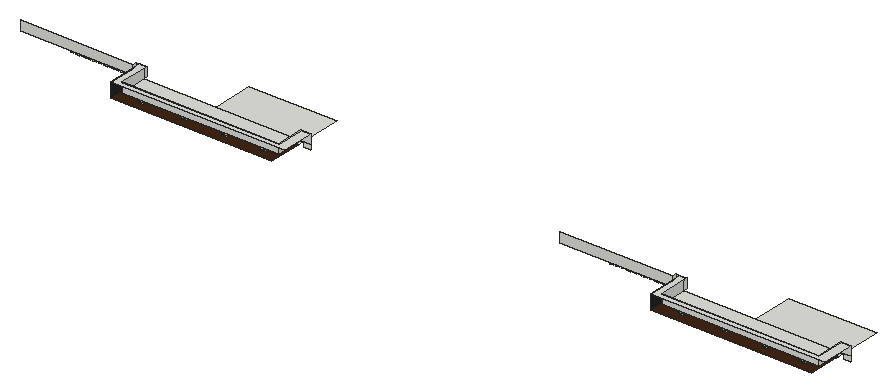
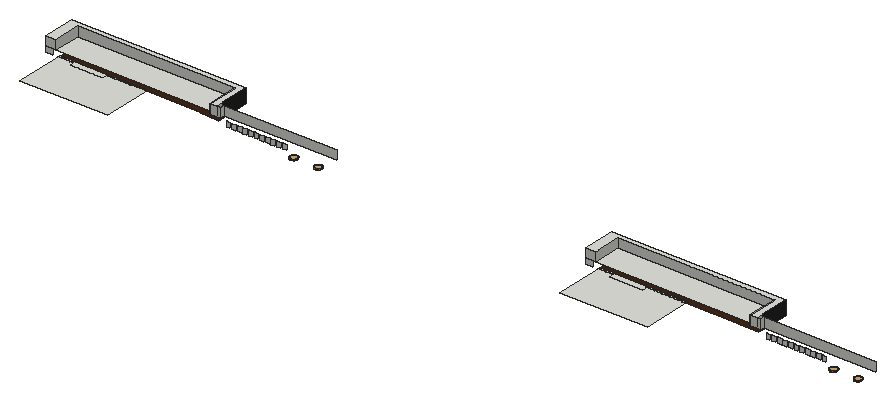
# SketchUp Ruby script. Lengths in inches.
U = 1.inch
M = Sketchup.active_model
def pt(a) = Geom::Point3d.new(a.map { |v| v * U })
def face(e, loops, mat)
  f = e.add_face(loops[0].map { |a| pt(a) })
  loops[1..].each { |l| e.add_face(l.map { |a| pt(a) }).erase! }
  f.material = f.back_material = mat if mat
  f
end
# faces: each face lists its corners as indices into pts; further lists are holes
def faces(e, pts, list, mat = nil) = list.each { |f| face(e, (f[0].is_a?(Array) ? f : [f]).map { |l| l.map { |i| pts[i] } }, mat) }
# xy, xz, yz: faces in a plane at the given z, y or x. An outline is a flat list of corners, or four numbers for a rectangle; further outlines are holes
def ring(l) = l.size == 4 ? [[l[0], l[1]], [l[2], l[1]], [l[2], l[3]], [l[0], l[3]]] : l.each_slice(2).to_a
def flat(e, list, mat, &to3) = list.each { |f| face(e, (f[0].is_a?(Array) ? f : [f]).map { |l| ring(l).map { |u, v| to3.(u, v) } }, mat) }
def xy(e, z, list, mat = nil) = flat(e, list, mat) { |x, y| [x, y, z] }
def xz(e, y, list, mat = nil) = flat(e, list, mat) { |x, z| [x, y, z] }
def yz(e, x, list, mat = nil) = flat(e, list, mat) { |y, z| [x, y, z] }
def lines(e, pts, list) = list.each { |a, b| e.add_line(pt(pts[a]), pt(pts[b])) }
# prism: a flat outline (further loops are holes) pulled along v
def prism(e, loops, v, mat = nil)
  f = face(e, loops, mat); d = Geom::Vector3d.new(v.map { |x| x * U })
  f.pushpull(f.normal.samedirection?(d) ? d.length : -d.length)
end
def box(e, o, s, mat = nil) = prism(e, [[o, [o[0] + s[0], o[1], o[2]], [o[0] + s[0], o[1] + s[1], o[2]], [o[0], o[1] + s[1], o[2]]]], [0, 0, s[2]], mat)
def at(x, y, z, deg = 0) = Geom::Transformation.translation(pt([x, y, z])) * Geom::Transformation.rotation(ORIGIN, Z_AXIS, deg.degrees)
def axes(o, x, y, z) = Geom::Transformation.new([*x, 0, *y, 0, *z, 0, *pt(o).to_a, 1])
def part(name) = M.definitions.add(name)
# library, detail: a bought-in or finely detailed component or shape, given as its bounding box
def library(name, o, s) = part(name).tap { |d| box(d.entities, o, s) }
def detail(e, o, s) = box(e.add_group.entities, o, s)
def put(e, d, t, mat = nil) = e.add_instance(d, t).tap { |i| i.material = mat if mat }
def group(e, t, mat = nil) = e.add_group.tap { |g| g.transformation = t; g.material = mat if mat }.entities
root = M.entities
M.materials.add("[Field Square Tile]").color = [211, 167, 108]
M.materials.add("[Granite Dark Gray]").color = [38, 37, 37]
M.materials.add("[Wood Veneer 01]").color = [66, 38, 20]
xy(root,380.5,[[2291.96,508.33,2297.38,511.08],[2297.38,508.33,2298.58,511.08],[2298.58,508.33,2304.01,511.08],[2304.01,508.33,2305.21,511.08],[2305.21,508.33,2310.63,511.08],
  [2310.63,508.33,2311.83,511.08],[2311.83,508.33,2317.26,511.08],[2317.26,508.33,2318.46,511.08],[2318.46,508.33,2323.88,511.08],[2323.88,508.33,2325.08,511.08],
  [2325.08,508.33,2330.51,511.08],[2330.51,508.33,2331.71,511.08],[2331.71,508.33,2337.13,511.08],[2337.13,508.33,2338.33,511.08],[2338.33,508.33,2343.76,511.08],
  [2343.76,508.33,2344.96,511.08],[2344.96,508.33,2350.38,511.08],[2350.38,508.33,2351.58,511.08],[2351.58,508.33,2357.01,511.08],[2357.01,508.33,2410.56,518.65],
  [2410.56,508.33,2415.98,511.08],[2415.98,508.33,2417.18,511.08],[2417.18,508.33,2422.61,511.08],[2422.61,508.33,2423.81,511.08],[2423.81,508.33,2429.23,511.08],
  [2429.23,508.33,2430.06,511.08],[2430.06,508.33,2434.04,511.08],[2434.04,508.33,2435.48,511.08],[3170.71,508.33,3176.13,511.08],[3176.13,508.33,3177.33,511.08],
  [3177.33,508.33,3182.76,511.08],[3182.76,508.33,3183.96,511.08],[3183.96,508.33,3189.38,511.08],[3189.38,508.33,3190.58,511.08],[3190.58,508.33,3196.01,511.08],
  [3196.01,508.33,3197.21,511.08],[3197.21,508.33,3202.63,511.08],[3202.63,508.33,3203.83,511.08],[3203.83,508.33,3209.26,511.08],[3209.26,508.33,3210.46,511.08],
  [3210.46,508.33,3215.88,511.08],[3215.88,508.33,3217.08,511.08],[3217.08,508.33,3222.51,511.08],[3222.51,508.33,3223.71,511.08],[3223.71,508.33,3229.13,511.08],
  [3229.13,508.33,3230.33,511.08],[3230.33,508.33,3235.76,511.08],[3235.76,508.33,3289.31,518.65],[3289.31,508.33,3294.73,511.08],[3294.73,508.33,3295.93,511.08],
  [3295.93,508.33,3301.36,511.08],[3301.36,508.33,3302.56,511.08],[3302.56,508.33,3307.98,511.08],[3307.98,508.33,3308.81,511.08],[3308.81,508.33,3312.79,511.08],
  [3312.79,508.33,3314.23,511.08],[2291.96,511.08,2291.96,589.83,2434.04,589.83,2434.04,511.08,2410.56,511.08,2410.56,518.65,2357.01,518.65,2357.01,511.08],[3170.71,511.08,3170.71,589.83,3312.79,589.83,3312.79,511.08,3289.31,511.08,3289.31,518.65,3235.76,518.65,3235.76,511.08]])
xy(root,380.5,[[[2172.48,458.5,2172.48,512.27,2202.28,512.27,2202.28,511.08,2291.96,511.08,2291.96,508.33,2434.04,508.33,2434.04,458.5],[2279.18,470.7,2280.73,470.9,2282.18,471.5,2283.42,472.46,2284.38,473.7,2284.98,475.15,2285.18,476.7,2284.98,478.25,2284.38,479.7,2283.42,480.94,2282.18,481.9,2280.73,482.49,2279.18,482.7,2277.63,482.49,2276.18,481.9,2274.9375,480.94,2273.99,479.7,2273.39,478.25,2273.18,476.7,2273.39,475.15,2273.99,473.7,2274.9375,472.46,2276.18,471.5,2277.63,470.9],[2346.46,470.7,2348.01,470.9,2349.46,471.5,2350.7,472.46,2351.66,473.7,2352.26,475.15,2352.46,476.7,2352.26,478.25,2351.66,479.7,2350.7,480.94,2349.46,481.9,2348.01,482.49,2346.46,482.7,2344.91,482.49,2343.46,481.9,2342.22,480.94,2341.26,479.7,2340.66,478.25,2340.46,476.7,2340.66,475.15,2341.26,473.7,2342.22,472.46,2343.46,471.5,2344.91,470.9],[2407.83,470.7,2409.39,470.9,2410.83,471.5,2412.08,472.46,2413.03,473.7,2413.63,475.15,2413.83,476.7,2413.63,478.25,2413.03,479.7,2412.08,480.94,2410.83,481.9,2409.39,482.49,2407.83,482.7,2406.28,482.49,2404.83,481.9,2403.59,480.94,2402.64,479.7,2402.04,478.25,2401.83,476.7,2402.04,475.15,2402.64,473.7,2403.59,472.46,2404.83,471.5,2406.28,470.9],[2209.72,470.7,2211.27,470.9,2212.72,471.5,2213.96,472.46,2214.91,473.7,2215.51,475.15,2215.72,476.7,2215.51,478.25,2214.91,479.7,2213.96,480.94,2212.72,481.9,2211.27,482.49,2209.72,482.7,2208.17,482.49,2206.72,481.9,2205.48,480.94,2204.52,479.7,2203.92,478.25,2203.72,476.7,2203.92,475.15,2204.52,473.7,2205.48,472.46,2206.72,471.5,2208.17,470.9]],[[3051.23,458.5,3051.23,512.27,3081.03,512.27,3081.03,511.08,3170.71,511.08,3170.71,508.33,3312.79,508.33,3312.79,458.5],[3157.93,470.7,3159.48,470.9,3160.93,471.5,3162.17,472.46,3163.13,473.7,3163.73,475.15,3163.93,476.7,3163.73,478.25,3163.13,479.7,3162.17,480.94,3160.93,481.9,3159.48,482.49,3157.93,482.7,3156.38,482.49,3154.93,481.9,3153.6875,480.94,3152.74,479.7,3152.14,478.25,3151.93,476.7,3152.14,475.15,3152.74,473.7,3153.6875,472.46,3154.93,471.5,3156.38,470.9],[3286.58,470.7,3288.14,470.9,3289.58,471.5,3290.83,472.46,3291.78,473.7,3292.38,475.15,3292.58,476.7,3292.38,478.25,3291.78,479.7,3290.83,480.94,3289.58,481.9,3288.14,482.49,3286.58,482.7,3285.03,482.49,3283.58,481.9,3282.34,480.94,3281.39,479.7,3280.79,478.25,3280.58,476.7,3280.79,475.15,3281.39,473.7,3282.34,472.46,3283.58,471.5,3285.03,470.9],[3088.47,470.7,3090.02,470.9,3091.47,471.5,3092.71,472.46,3093.66,473.7,3094.26,475.15,3094.47,476.7,3094.26,478.25,3093.66,479.7,3092.71,480.94,3091.47,481.9,3090.02,482.49,3088.47,482.7,3086.92,482.49,3085.47,481.9,3084.23,480.94,3083.27,479.7,3082.67,478.25,3082.47,476.7,3082.67,475.15,3083.27,473.7,3084.23,472.46,3085.47,471.5,3086.92,470.9],[3225.21,470.7,3226.76,470.9,3228.21,471.5,3229.45,472.46,3230.41,473.7,3231.01,475.15,3231.21,476.7,3231.01,478.25,3230.41,479.7,3229.45,480.94,3228.21,481.9,3226.76,482.49,3225.21,482.7,3223.66,482.49,3222.21,481.9,3220.97,480.94,3220.01,479.7,3219.41,478.25,3219.21,476.7,3219.41,475.15,3220.01,473.7,3220.97,472.46,3222.21,471.5,3223.66,470.9]]],"[Wood Veneer 01]")
xy(root,381.8125,[[2209.72,470.7,2208.17,470.9,2206.72,471.5,2205.48,472.46,2204.52,473.7,2203.92,475.15,2203.72,476.7,2203.92,478.25,2204.52,479.7,2205.48,480.94,2206.72,481.9,2208.17,482.49,2209.72,482.7,2211.27,482.49,2212.72,481.9,2213.96,480.94,2214.91,479.7,2215.51,478.25,2215.72,476.7,2215.51,475.15,2214.91,473.7,2213.96,472.46,2212.72,471.5,2211.27,470.9],[2279.18,470.7,2277.63,470.9,2276.18,471.5,2274.9375,472.46,2273.99,473.7,2273.39,475.15,2273.18,476.7,2273.39,478.25,2273.99,479.7,2274.9375,480.94,2276.18,481.9,2277.63,482.49,2279.18,482.7,2280.73,482.49,2282.18,481.9,2283.42,480.94,2284.38,479.7,2284.98,478.25,2285.18,476.7,2284.98,475.15,2284.38,473.7,2283.42,472.46,2282.18,471.5,2280.73,470.9],[2346.46,470.7,2344.91,470.9,2343.46,471.5,2342.22,472.46,2341.26,473.7,2340.66,475.15,2340.46,476.7,2340.66,478.25,2341.26,479.7,2342.22,480.94,2343.46,481.9,2344.91,482.49,2346.46,482.7,2348.01,482.49,2349.46,481.9,2350.7,480.94,2351.66,479.7,2352.26,478.25,2352.46,476.7,2352.26,475.15,2351.66,473.7,2350.7,472.46,2349.46,471.5,2348.01,470.9],[2407.83,470.7,2406.28,470.9,2404.83,471.5,2403.59,472.46,2402.64,473.7,2402.04,475.15,2401.83,476.7,2402.04,478.25,2402.64,479.7,2403.59,480.94,2404.83,481.9,2406.28,482.49,2407.83,482.7,2409.39,482.49,2410.83,481.9,2412.08,480.94,2413.03,479.7,2413.63,478.25,2413.83,476.7,2413.63,475.15,2413.03,473.7,2412.08,472.46,2410.83,471.5,2409.39,470.9],[3088.47,470.7,3086.92,470.9,3085.47,471.5,3084.23,472.46,3083.27,473.7,3082.67,475.15,3082.47,476.7,3082.67,478.25,3083.27,479.7,3084.23,480.94,3085.47,481.9,3086.92,482.49,3088.47,482.7,3090.02,482.49,3091.47,481.9,3092.71,480.94,3093.66,479.7,3094.26,478.25,3094.47,476.7,3094.26,475.15,3093.66,473.7,3092.71,472.46,3091.47,471.5,3090.02,470.9],
  [3157.93,470.7,3156.38,470.9,3154.93,471.5,3153.6875,472.46,3152.74,473.7,3152.14,475.15,3151.93,476.7,3152.14,478.25,3152.74,479.7,3153.6875,480.94,3154.93,481.9,3156.38,482.49,3157.93,482.7,3159.48,482.49,3160.93,481.9,3162.17,480.94,3163.13,479.7,3163.73,478.25,3163.93,476.7,3163.73,475.15,3163.13,473.7,3162.17,472.46,3160.93,471.5,3159.48,470.9],[3225.21,470.7,3223.66,470.9,3222.21,471.5,3220.97,472.46,3220.01,473.7,3219.41,475.15,3219.21,476.7,3219.41,478.25,3220.01,479.7,3220.97,480.94,3222.21,481.9,3223.66,482.49,3225.21,482.7,3226.76,482.49,3228.21,481.9,3229.45,480.94,3230.41,479.7,3231.01,478.25,3231.21,476.7,3231.01,475.15,3230.41,473.7,3229.45,472.46,3228.21,471.5,3226.76,470.9],[3286.58,470.7,3285.03,470.9,3283.58,471.5,3282.34,472.46,3281.39,473.7,3280.79,475.15,3280.58,476.7,3280.79,478.25,3281.39,479.7,3282.34,480.94,3283.58,481.9,3285.03,482.49,3286.58,482.7,3288.14,482.49,3289.58,481.9,3290.83,480.94,3291.78,479.7,3292.38,478.25,3292.58,476.7,3292.38,475.15,3291.78,473.7,3290.83,472.46,3289.58,471.5,3288.14,470.9]],"[Field Square Tile]")
xy(root,381.875,[[1998.33,523.51,1996.77,523.54,1995.26,523.98,1993.92,524.79,1992.84,525.92,1992.08,527.29,1991.71,528.8125,1991.74,530.375,1992.18,531.88,1992.99,533.22,1994.12,534.31,1995.49,535.06,1997.01,535.43,1998.58,535.4,2000.08,534.96,2001.42,534.15,2002.51,533.02,2003.26,531.65,2003.64,530.13,2003.6,528.5625,2003.17,527.06,2002.36,525.72,2001.23,524.64,1999.85,523.88],[2038.08,523.51,2036.52,523.54,2035.01,523.98,2033.67,524.79,2032.59,525.92,2031.83,527.29,2031.46,528.8125,2031.49,530.375,2031.93,531.88,2032.74,533.22,2033.87,534.31,2035.24,535.06,2036.76,535.43,2038.33,535.4,2039.83,534.96,2041.17,534.15,2042.26,533.02,2043.01,531.65,2043.39,530.13,2043.35,528.5625,2042.92,527.06,2042.11,525.72,2040.98,524.64,2039.6,523.88],[2877.08,523.51,2875.52,523.54,2874.01,523.98,2872.67,524.79,2871.59,525.92,2870.83,527.29,2870.46,528.8125,2870.49,530.375,2870.93,531.88,2871.74,533.22,2872.87,534.31,2874.24,535.06,2875.76,535.43,2877.33,535.4,2878.83,534.96,2880.17,534.15,2881.26,533.02,2882.01,531.65,2882.39,530.13,2882.35,528.5625,2881.92,527.06,2881.11,525.72,2879.98,524.64,2878.6,523.88],[2916.83,523.51,2915.27,523.54,2913.76,523.98,2912.42,524.79,2911.34,525.92,2910.58,527.29,2910.21,528.8125,2910.24,530.375,2910.68,531.88,2911.49,533.22,2912.62,534.31,2913.99,535.06,2915.51,535.43,2917.08,535.4,2918.58,534.96,2919.92,534.15,2921.01,533.02,2921.76,531.65,2922.14,530.13,2922.1,528.5625,2921.67,527.06,2920.86,525.72,2919.73,524.64,2918.35,523.88]],"[Field Square Tile]")
xy(root,388.625,[[2183.1875,466.05,2439.68,511.08],[3061.9375,466.05,3318.43,511.08]])
xy(root,403.8125,[[2172.48,458.5,2455.66,458.5,2455.66,511.08,2439.68,511.08,2439.68,466.05,2183.1875,466.05,2183.1875,517.43,2172.48,517.43],[3051.23,458.5,3334.41,458.5,3334.41,511.08,3318.43,511.08,3318.43,466.05,3061.9375,466.05,3061.9375,517.43,3051.23,517.43]])
xz(root,466.05,[[2183.1875,388.625,2439.68,403.8125],[3061.9375,388.625,3318.43,403.8125]])
xz(root,510.87,[[1982.81,388.625,2166.13,403.8125],[2861.56,388.625,3044.88,403.8125]])
xz(root,511.08,[[2443.85,380.5,2455.66,388.625],[3322.6,380.5,3334.41,388.625],[2439.68,388.625,2455.66,403.8125],[3318.43,388.625,3334.41,403.8125]])
xz(root,517.43,[[2166.13,388.625,2172.48,403.8125],[2172.48,388.625,2183.1875,403.8125],[3044.88,388.625,3051.23,403.8125],[3051.23,388.625,3061.9375,403.8125]])
xz(root,519.43,[[2057.43,380.5,2063.68,388.625],[2066.56,380.5,2072.81,388.625],[2075.68,380.5,2081.93,388.625],[2084.81,380.5,2091.06,388.625],[2093.93,380.5,2100.18,388.625],
  [2103.06,380.5,2109.31,388.625],[2112.18,380.5,2118.43,388.625],[2121.31,380.5,2127.56,388.625],[2130.43,380.5,2136.68,388.625],[2139.56,380.5,2145.81,388.625],
  [2148.68,380.5,2154.93,388.625],[2936.18,380.5,2942.43,388.625],[2945.31,380.5,2951.56,388.625],[2954.43,380.5,2960.68,388.625],[2963.56,380.5,2969.81,388.625],
  [2972.68,380.5,2978.93,388.625],[2981.81,380.5,2988.06,388.625],[2990.93,380.5,2997.18,388.625],[3000.06,380.5,3006.31,388.625],[3009.18,380.5,3015.43,388.625],
  [3018.31,380.5,3024.56,388.625],[3027.43,380.5,3033.68,388.625]])
yz(root,2166.13,[[510.87,388.625,517.43,403.8125]])
yz(root,2172.48,[[458.5,380.5,504.52,403.8125]],"[Granite Dark Gray]")
yz(root,2183.1875,[[466.05,388.625,511.08,403.8125],[511.08,388.625,517.43,403.8125]])
yz(root,2439.68,[[466.05,388.625,511.08,403.8125]])
yz(root,3044.88,[[510.87,388.625,517.43,403.8125]])
yz(root,3051.23,[[458.5,380.5,504.52,403.8125]],"[Granite Dark Gray]")
yz(root,3061.9375,[[466.05,388.625,511.08,403.8125],[511.08,388.625,517.43,403.8125]])
yz(root,3318.43,[[466.05,388.625,511.08,403.8125]])
p = [[2209.72,470.7,380.5],[2208.17,470.9,380.5],[2208.17,470.9,381.8125],[2209.72,470.7,381.8125],[2211.27,470.9,380.5],[2211.27,470.9,381.8125],
  [2279.18,470.7,380.5],[2277.63,470.9,380.5],[2277.63,470.9,381.8125],[2279.18,470.7,381.8125],[2280.73,470.9,380.5],[2280.73,470.9,381.8125],
  [2346.46,470.7,380.5],[2344.91,470.9,380.5],[2344.91,470.9,381.8125],[2346.46,470.7,381.8125],[2348.01,470.9,380.5],[2348.01,470.9,381.8125],
  [2407.83,470.7,380.5],[2406.28,470.9,380.5],[2406.28,470.9,381.8125],[2407.83,470.7,381.8125],[2409.39,470.9,380.5],[2409.39,470.9,381.8125],
  [3088.47,470.7,380.5],[3086.92,470.9,380.5],[3086.92,470.9,381.8125],[3088.47,470.7,381.8125],[3090.02,470.9,380.5],[3090.02,470.9,381.8125],
  [3157.93,470.7,380.5],[3156.38,470.9,380.5],[3156.38,470.9,381.8125],[3157.93,470.7,381.8125],[3159.48,470.9,380.5],[3159.48,470.9,381.8125],
  [3225.21,470.7,380.5],[3223.66,470.9,380.5],[3223.66,470.9,381.8125],[3225.21,470.7,381.8125],[3226.76,470.9,380.5],[3226.76,470.9,381.8125],
  [3286.58,470.7,380.5],[3285.03,470.9,380.5],[3285.03,470.9,381.8125],[3286.58,470.7,381.8125],[3288.14,470.9,380.5],[3288.14,470.9,381.8125],
  [2206.72,471.5,380.5],[2206.72,471.5,381.8125],[2212.72,471.5,380.5],[2212.72,471.5,381.8125],[2276.18,471.5,380.5],[2276.18,471.5,381.8125],
  [2282.18,471.5,380.5],[2282.18,471.5,381.8125],[2343.46,471.5,380.5],[2343.46,471.5,381.8125],[2349.46,471.5,380.5],[2349.46,471.5,381.8125],
  [2404.83,471.5,380.5],[2404.83,471.5,381.8125],[2410.83,471.5,380.5],[2410.83,471.5,381.8125],[3085.47,471.5,380.5],[3085.47,471.5,381.8125],
  [3091.47,471.5,380.5],[3091.47,471.5,381.8125],[3154.93,471.5,380.5],[3154.93,471.5,381.8125],[3160.93,471.5,380.5],[3160.93,471.5,381.8125],
  [3222.21,471.5,380.5],[3222.21,471.5,381.8125],[3228.21,471.5,380.5],[3228.21,471.5,381.8125],[3283.58,471.5,380.5],[3283.58,471.5,381.8125],
  [3289.58,471.5,380.5],[3289.58,471.5,381.8125],[2205.48,472.46,380.5],[2205.48,472.46,381.8125],[2213.96,472.46,380.5],[2213.96,472.46,381.8125],
  [2274.9375,472.46,380.5],[2274.9375,472.46,381.8125],[2283.42,472.46,380.5],[2283.42,472.46,381.8125],[2342.22,472.46,380.5],[2342.22,472.46,381.8125],
  [2350.7,472.46,380.5],[2350.7,472.46,381.8125],[2403.59,472.46,380.5],[2403.59,472.46,381.8125],[2412.08,472.46,380.5],[2412.08,472.46,381.8125],
  [3084.23,472.46,380.5],[3084.23,472.46,381.8125],[3092.71,472.46,380.5],[3092.71,472.46,381.8125],[3153.6875,472.46,380.5],[3153.6875,472.46,381.8125],
  [3162.17,472.46,380.5],[3162.17,472.46,381.8125],[3220.97,472.46,380.5],[3220.97,472.46,381.8125],[3229.45,472.46,380.5],[3229.45,472.46,381.8125],
  [3282.34,472.46,380.5],[3282.34,472.46,381.8125],[3290.83,472.46,380.5],[3290.83,472.46,381.8125],[2204.52,473.7,380.5],[2204.52,473.7,381.8125],
  [2214.91,473.7,380.5],[2214.91,473.7,381.8125],[2273.99,473.7,380.5],[2273.99,473.7,381.8125],[2284.38,473.7,380.5],[2284.38,473.7,381.8125],
  [2341.26,473.7,380.5],[2341.26,473.7,381.8125],[2351.66,473.7,380.5],[2351.66,473.7,381.8125],[2402.64,473.7,380.5],[2402.64,473.7,381.8125],
  [2413.03,473.7,380.5],[2413.03,473.7,381.8125],[3083.27,473.7,380.5],[3083.27,473.7,381.8125],[3093.66,473.7,380.5],[3093.66,473.7,381.8125],
  [3152.74,473.7,380.5],[3152.74,473.7,381.8125],[3163.13,473.7,380.5],[3163.13,473.7,381.8125],[3220.01,473.7,380.5],[3220.01,473.7,381.8125],
  [3230.41,473.7,380.5],[3230.41,473.7,381.8125],[3281.39,473.7,380.5],[3281.39,473.7,381.8125],[3291.78,473.7,380.5],[3291.78,473.7,381.8125],
  [2203.92,475.15,380.5],[2203.92,475.15,381.8125],[2215.51,475.15,380.5],[2215.51,475.15,381.8125],[2273.39,475.15,380.5],[2273.39,475.15,381.8125],
  [2284.98,475.15,380.5],[2284.98,475.15,381.8125],[2340.66,475.15,380.5],[2340.66,475.15,381.8125],[2352.26,475.15,380.5],[2352.26,475.15,381.8125],
  [2402.04,475.15,380.5],[2402.04,475.15,381.8125],[2413.63,475.15,380.5],[2413.63,475.15,381.8125],[3082.67,475.15,380.5],[3082.67,475.15,381.8125],
  [3094.26,475.15,380.5],[3094.26,475.15,381.8125],[3152.14,475.15,380.5],[3152.14,475.15,381.8125],[3163.73,475.15,380.5],[3163.73,475.15,381.8125],
  [3219.41,475.15,380.5],[3219.41,475.15,381.8125],[3231.01,475.15,380.5],[3231.01,475.15,381.8125],[3280.79,475.15,380.5],[3280.79,475.15,381.8125],
  [3292.38,475.15,380.5],[3292.38,475.15,381.8125],[2203.72,476.7,380.5],[2203.72,476.7,381.8125],[2215.72,476.7,380.5],[2215.72,476.7,381.8125],
  [2273.18,476.7,380.5],[2273.18,476.7,381.8125],[2285.18,476.7,380.5],[2285.18,476.7,381.8125],[2340.46,476.7,380.5],[2340.46,476.7,381.8125],
  [2352.46,476.7,380.5],[2352.46,476.7,381.8125],[2401.83,476.7,380.5],[2401.83,476.7,381.8125],[2413.83,476.7,380.5],[2413.83,476.7,381.8125],
  [3082.47,476.7,380.5],[3082.47,476.7,381.8125],[3094.47,476.7,380.5],[3094.47,476.7,381.8125],[3151.93,476.7,380.5],[3151.93,476.7,381.8125],
  [3163.93,476.7,380.5],[3163.93,476.7,381.8125],[3219.21,476.7,380.5],[3219.21,476.7,381.8125],[3231.21,476.7,380.5],[3231.21,476.7,381.8125],
  [3280.58,476.7,380.5],[3280.58,476.7,381.8125],[3292.58,476.7,380.5],[3292.58,476.7,381.8125],[2203.92,478.25,380.5],[2203.92,478.25,381.8125],
  [2215.51,478.25,380.5],[2215.51,478.25,381.8125],[2273.39,478.25,380.5],[2273.39,478.25,381.8125],[2284.98,478.25,380.5],[2284.98,478.25,381.8125],
  [2340.66,478.25,380.5],[2340.66,478.25,381.8125],[2352.26,478.25,380.5],[2352.26,478.25,381.8125],[2402.04,478.25,380.5],[2402.04,478.25,381.8125],
  [2413.63,478.25,380.5],[2413.63,478.25,381.8125],[3082.67,478.25,380.5],[3082.67,478.25,381.8125],[3094.26,478.25,380.5],[3094.26,478.25,381.8125],
  [3152.14,478.25,380.5],[3152.14,478.25,381.8125],[3163.73,478.25,380.5],[3163.73,478.25,381.8125],[3219.41,478.25,380.5],[3219.41,478.25,381.8125],
  [3231.01,478.25,380.5],[3231.01,478.25,381.8125],[3280.79,478.25,380.5],[3280.79,478.25,381.8125],[3292.38,478.25,380.5],[3292.38,478.25,381.8125],
  [2204.52,479.7,380.5],[2204.52,479.7,381.8125],[2214.91,479.7,380.5],[2214.91,479.7,381.8125],[2273.99,479.7,380.5],[2273.99,479.7,381.8125],
  [2284.38,479.7,380.5],[2284.38,479.7,381.8125],[2341.26,479.7,380.5],[2341.26,479.7,381.8125],[2351.66,479.7,380.5],[2351.66,479.7,381.8125],
  [2402.64,479.7,380.5],[2402.64,479.7,381.8125],[2413.03,479.7,380.5],[2413.03,479.7,381.8125],[3083.27,479.7,380.5],[3083.27,479.7,381.8125],
  [3093.66,479.7,380.5],[3093.66,479.7,381.8125],[3152.74,479.7,380.5],[3152.74,479.7,381.8125],[3163.13,479.7,380.5],[3163.13,479.7,381.8125],
  [3220.01,479.7,380.5],[3220.01,479.7,381.8125],[3230.41,479.7,380.5],[3230.41,479.7,381.8125],[3281.39,479.7,380.5],[3281.39,479.7,381.8125],
  [3291.78,479.7,380.5],[3291.78,479.7,381.8125],[2205.48,480.94,380.5],[2205.48,480.94,381.8125],[2213.96,480.94,380.5],[2213.96,480.94,381.8125],
  [2274.9375,480.94,380.5],[2274.9375,480.94,381.8125],[2283.42,480.94,380.5],[2283.42,480.94,381.8125],[2342.22,480.94,380.5],[2342.22,480.94,381.8125],
  [2350.7,480.94,380.5],[2350.7,480.94,381.8125],[2403.59,480.94,380.5],[2403.59,480.94,381.8125],[2412.08,480.94,380.5],[2412.08,480.94,381.8125],
  [3084.23,480.94,380.5],[3084.23,480.94,381.8125],[3092.71,480.94,380.5],[3092.71,480.94,381.8125],[3153.6875,480.94,380.5],[3153.6875,480.94,381.8125],
  [3162.17,480.94,380.5],[3162.17,480.94,381.8125],[3220.97,480.94,380.5],[3220.97,480.94,381.8125],[3229.45,480.94,380.5],[3229.45,480.94,381.8125],
  [3282.34,480.94,380.5],[3282.34,480.94,381.8125],[3290.83,480.94,380.5],[3290.83,480.94,381.8125],[2206.72,481.9,380.5],[2206.72,481.9,381.8125],
  [2212.72,481.9,380.5],[2212.72,481.9,381.8125],[2276.18,481.9,380.5],[2276.18,481.9,381.8125],[2282.18,481.9,380.5],[2282.18,481.9,381.8125],
  [2343.46,481.9,380.5],[2343.46,481.9,381.8125],[2349.46,481.9,380.5],[2349.46,481.9,381.8125],[2404.83,481.9,380.5],[2404.83,481.9,381.8125],
  [2410.83,481.9,380.5],[2410.83,481.9,381.8125],[3085.47,481.9,380.5],[3085.47,481.9,381.8125],[3091.47,481.9,380.5],[3091.47,481.9,381.8125],
  [3154.93,481.9,380.5],[3154.93,481.9,381.8125],[3160.93,481.9,380.5],[3160.93,481.9,381.8125],[3222.21,481.9,380.5],[3222.21,481.9,381.8125],
  [3228.21,481.9,380.5],[3228.21,481.9,381.8125],[3283.58,481.9,380.5],[3283.58,481.9,381.8125],[3289.58,481.9,380.5],[3289.58,481.9,381.8125],
  [2208.17,482.49,380.5],[2208.17,482.49,381.8125],[2211.27,482.49,380.5],[2211.27,482.49,381.8125],[2277.63,482.49,380.5],[2277.63,482.49,381.8125],
  [2280.73,482.49,380.5],[2280.73,482.49,381.8125],[2344.91,482.49,380.5],[2344.91,482.49,381.8125],[2348.01,482.49,380.5],[2348.01,482.49,381.8125],
  [2406.28,482.49,380.5],[2406.28,482.49,381.8125],[2409.39,482.49,380.5],[2409.39,482.49,381.8125],[3086.92,482.49,380.5],[3086.92,482.49,381.8125],
  [3090.02,482.49,380.5],[3090.02,482.49,381.8125],[3156.38,482.49,380.5],[3156.38,482.49,381.8125],[3159.48,482.49,380.5],[3159.48,482.49,381.8125],
  [3223.66,482.49,380.5],[3223.66,482.49,381.8125],[3226.76,482.49,380.5],[3226.76,482.49,381.8125],[3285.03,482.49,380.5],[3285.03,482.49,381.8125],
  [3288.14,482.49,380.5],[3288.14,482.49,381.8125],[2209.72,482.7,380.5],[2209.72,482.7,381.8125],[2279.18,482.7,380.5],[2279.18,482.7,381.8125],
  [2346.46,482.7,380.5],[2346.46,482.7,381.8125],[2407.83,482.7,380.5],[2407.83,482.7,381.8125],[3088.47,482.7,380.5],[3088.47,482.7,381.8125],
  [3157.93,482.7,380.5],[3157.93,482.7,381.8125],[3225.21,482.7,380.5],[3225.21,482.7,381.8125],[3286.58,482.7,380.5],[3286.58,482.7,381.8125],
  [1996.77,523.54,380.5],[1995.26,523.98,380.5],[1995.26,523.98,381.875],[1996.77,523.54,381.875],[1998.33,523.51,380.5],[1998.33,523.51,381.875],
  [1999.85,523.88,380.5],[1999.85,523.88,381.875],[2036.52,523.54,380.5],[2035.01,523.98,380.5],[2035.01,523.98,381.875],[2036.52,523.54,381.875],
  [2038.08,523.51,380.5],[2038.08,523.51,381.875],[2039.6,523.88,380.5],[2039.6,523.88,381.875],[2875.52,523.54,380.5],[2874.01,523.98,380.5],
  [2874.01,523.98,381.875],[2875.52,523.54,381.875],[2877.08,523.51,380.5],[2877.08,523.51,381.875],[2878.6,523.88,380.5],[2878.6,523.88,381.875],
  [2915.27,523.54,380.5],[2913.76,523.98,380.5],[2913.76,523.98,381.875],[2915.27,523.54,381.875],[2916.83,523.51,380.5],[2916.83,523.51,381.875],
  [2918.35,523.88,380.5],[2918.35,523.88,381.875],[2001.23,524.64,380.5],[2001.23,524.64,381.875],[2040.98,524.64,380.5],[2040.98,524.64,381.875],
  [2879.98,524.64,380.5],[2879.98,524.64,381.875],[2919.73,524.64,380.5],[2919.73,524.64,381.875],[1993.92,524.79,380.5],[1993.92,524.79,381.875],
  [2033.67,524.79,380.5],[2033.67,524.79,381.875],[2872.67,524.79,380.5],[2872.67,524.79,381.875],[2912.42,524.79,380.5],[2912.42,524.79,381.875],
  [2002.36,525.72,380.5],[2002.36,525.72,381.875],[2042.11,525.72,380.5],[2042.11,525.72,381.875],[2881.11,525.72,380.5],[2881.11,525.72,381.875],
  [2920.86,525.72,380.5],[2920.86,525.72,381.875],[1992.84,525.92,380.5],[1992.84,525.92,381.875],[2032.59,525.92,380.5],[2032.59,525.92,381.875],
  [2871.59,525.92,380.5],[2871.59,525.92,381.875],[2911.34,525.92,380.5],[2911.34,525.92,381.875],[2003.17,527.06,380.5],[2003.17,527.06,381.875],
  [2042.92,527.06,380.5],[2042.92,527.06,381.875],[2881.92,527.06,380.5],[2881.92,527.06,381.875],[2921.67,527.06,380.5],[2921.67,527.06,381.875],
  [1992.08,527.29,380.5],[1992.08,527.29,381.875],[2031.83,527.29,380.5],[2031.83,527.29,381.875],[2870.83,527.29,380.5],[2870.83,527.29,381.875],
  [2910.58,527.29,380.5],[2910.58,527.29,381.875],[2003.6,528.5625,380.5],[2003.6,528.5625,381.875],[2043.35,528.5625,380.5],[2043.35,528.5625,381.875],
  [2882.35,528.5625,380.5],[2882.35,528.5625,381.875],[2922.1,528.5625,380.5],[2922.1,528.5625,381.875],[1991.71,528.8125,380.5],[1991.71,528.8125,381.875],
  [2031.46,528.8125,380.5],[2031.46,528.8125,381.875],[2870.46,528.8125,380.5],[2870.46,528.8125,381.875],[2910.21,528.8125,380.5],[2910.21,528.8125,381.875],
  [2003.64,530.13,380.5],[2003.64,530.13,381.875],[2043.39,530.13,380.5],[2043.39,530.13,381.875],[2882.39,530.13,380.5],[2882.39,530.13,381.875],
  [2922.14,530.13,380.5],[2922.14,530.13,381.875],[1991.74,530.375,380.5],[1991.74,530.375,381.875],[2031.49,530.375,380.5],[2031.49,530.375,381.875],
  [2870.49,530.375,380.5],[2870.49,530.375,381.875],[2910.24,530.375,380.5],[2910.24,530.375,381.875],[2003.26,531.65,380.5],[2003.26,531.65,381.875],
  [2043.01,531.65,380.5],[2043.01,531.65,381.875],[2882.01,531.65,380.5],[2882.01,531.65,381.875],[2921.76,531.65,380.5],[2921.76,531.65,381.875],
  [1992.18,531.88,380.5],[1992.18,531.88,381.875],[2031.93,531.88,380.5],[2031.93,531.88,381.875],[2870.93,531.88,380.5],[2870.93,531.88,381.875],
  [2910.68,531.88,380.5],[2910.68,531.88,381.875],[2002.51,533.02,380.5],[2002.51,533.02,381.875],[2042.26,533.02,380.5],[2042.26,533.02,381.875],
  [2881.26,533.02,380.5],[2881.26,533.02,381.875],[2921.01,533.02,380.5],[2921.01,533.02,381.875],[1992.99,533.22,380.5],[1992.99,533.22,381.875],
  [2032.74,533.22,380.5],[2032.74,533.22,381.875],[2871.74,533.22,380.5],[2871.74,533.22,381.875],[2911.49,533.22,380.5],[2911.49,533.22,381.875],
  [2001.42,534.15,380.5],[2001.42,534.15,381.875],[2041.17,534.15,380.5],[2041.17,534.15,381.875],[2880.17,534.15,380.5],[2880.17,534.15,381.875],
  [2919.92,534.15,380.5],[2919.92,534.15,381.875],[1994.12,534.31,380.5],[1994.12,534.31,381.875],[2033.87,534.31,380.5],[2033.87,534.31,381.875],
  [2872.87,534.31,380.5],[2872.87,534.31,381.875],[2912.62,534.31,380.5],[2912.62,534.31,381.875],[2000.08,534.96,380.5],[2000.08,534.96,381.875],
  [2039.83,534.96,380.5],[2039.83,534.96,381.875],[2878.83,534.96,380.5],[2878.83,534.96,381.875],[2918.58,534.96,380.5],[2918.58,534.96,381.875],
  [1995.49,535.06,380.5],[1995.49,535.06,381.875],[2035.24,535.06,380.5],[2035.24,535.06,381.875],[2874.24,535.06,380.5],[2874.24,535.06,381.875],
  [2913.99,535.06,380.5],[2913.99,535.06,381.875],[1998.58,535.4,380.5],[1998.58,535.4,381.875],[2038.33,535.4,380.5],[2038.33,535.4,381.875],
  [2877.33,535.4,380.5],[2877.33,535.4,381.875],[2917.08,535.4,380.5],[2917.08,535.4,381.875],[1997.01,535.43,380.5],[1997.01,535.43,381.875],
  [2036.76,535.43,380.5],[2036.76,535.43,381.875],[2875.76,535.43,380.5],[2875.76,535.43,381.875],[2915.51,535.43,380.5],[2915.51,535.43,381.875],
  [2172.5,468.31,380.5],[2172.48,458.5,380.5],[3051.25,468.31,380.5],[3051.23,458.5,380.5]]
faces(root,p,[[0,1,2,3],[4,0,3,5],[6,7,8,9],[10,6,9,11],[12,13,14,15],[16,12,15,17],[18,19,20,21],[22,18,21,23],
  [24,25,26,27],[28,24,27,29],[30,31,32,33],[34,30,33,35],[36,37,38,39],[40,36,39,41],[42,43,44,45],[46,42,45,47],
  [1,48,49,2],[50,4,5,51],[7,52,53,8],[54,10,11,55],[13,56,57,14],[58,16,17,59],[19,60,61,20],[62,22,23,63],
  [25,64,65,26],[66,28,29,67],[31,68,69,32],[70,34,35,71],[37,72,73,38],[74,40,41,75],[43,76,77,44],[78,46,47,79],
  [48,80,81,49],[82,50,51,83],[52,84,85,53],[86,54,55,87],[56,88,89,57],[90,58,59,91],[60,92,93,61],[94,62,63,95],
  [64,96,97,65],[98,66,67,99],[68,100,101,69],[102,70,71,103],[72,104,105,73],[106,74,75,107],[76,108,109,77],[110,78,79,111],
  [80,112,113,81],[114,82,83,115],[84,116,117,85],[118,86,87,119],[88,120,121,89],[122,90,91,123],[92,124,125,93],[126,94,95,127],
  [96,128,129,97],[130,98,99,131],[100,132,133,101],[134,102,103,135],[104,136,137,105],[138,106,107,139],[108,140,141,109],[142,110,111,143],
  [112,144,145,113],[146,114,115,147],[116,148,149,117],[150,118,119,151],[120,152,153,121],[154,122,123,155],[124,156,157,125],[158,126,127,159],
  [128,160,161,129],[162,130,131,163],[132,164,165,133],[166,134,135,167],[136,168,169,137],[170,138,139,171],[140,172,173,141],[174,142,143,175],
  [144,176,177,145],[178,146,147,179],[148,180,181,149],[182,150,151,183],[152,184,185,153],[186,154,155,187],[156,188,189,157],[190,158,159,191],
  [160,192,193,161],[194,162,163,195],[164,196,197,165],[198,166,167,199],[168,200,201,169],[202,170,171,203],[172,204,205,173],[206,174,175,207],
  [176,208,209,177],[210,178,179,211],[180,212,213,181],[214,182,183,215],[184,216,217,185],[218,186,187,219],[188,220,221,189],[222,190,191,223],
  [192,224,225,193],[226,194,195,227],[196,228,229,197],[230,198,199,231],[200,232,233,201],[234,202,203,235],[204,236,237,205],[238,206,207,239],
  [208,240,241,209],[242,210,211,243],[212,244,245,213],[246,214,215,247],[216,248,249,217],[250,218,219,251],[220,252,253,221],[254,222,223,255],
  [224,256,257,225],[258,226,227,259],[228,260,261,229],[262,230,231,263],[232,264,265,233],[266,234,235,267],[236,268,269,237],[270,238,239,271],
  [240,272,273,241],[274,242,243,275],[244,276,277,245],[278,246,247,279],[248,280,281,249],[282,250,251,283],[252,284,285,253],[286,254,255,287],
  [256,288,289,257],[290,258,259,291],[260,292,293,261],[294,262,263,295],[264,296,297,265],[298,266,267,299],[268,300,301,269],[302,270,271,303],
  [272,304,305,273],[306,274,275,307],[276,308,309,277],[310,278,279,311],[280,312,313,281],[314,282,283,315],[284,316,317,285],[318,286,287,319],
  [288,320,321,289],[322,290,291,323],[292,324,325,293],[326,294,295,327],[296,328,329,297],[330,298,299,331],[300,332,333,301],[334,302,303,335],
  [304,336,337,305],[338,306,307,339],[308,340,341,309],[342,310,311,343],[312,344,345,313],[346,314,315,347],[316,348,349,317],[350,318,319,351],
  [320,352,353,321],[354,322,323,355],[324,356,357,325],[358,326,327,359],[328,360,361,329],[362,330,331,363],[332,364,365,333],[366,334,335,367],
  [336,368,369,337],[368,338,339,369],[340,370,371,341],[370,342,343,371],[344,372,373,345],[372,346,347,373],[348,374,375,349],[374,350,351,375],
  [352,376,377,353],[376,354,355,377],[356,378,379,357],[378,358,359,379],[360,380,381,361],[380,362,363,381],[364,382,383,365],[382,366,367,383],
  [384,385,386,387],[388,384,387,389],[390,388,389,391],[392,393,394,395],[396,392,395,397],[398,396,397,399],[400,401,402,403],[404,400,403,405],
  [406,404,405,407],[408,409,410,411],[412,408,411,413],[414,412,413,415],[416,390,391,417],[418,398,399,419],[420,406,407,421],[422,414,415,423],
  [385,424,425,386],[393,426,427,394],[401,428,429,402],[409,430,431,410],[432,416,417,433],[434,418,419,435],[436,420,421,437],[438,422,423,439],
  [424,440,441,425],[426,442,443,427],[428,444,445,429],[430,446,447,431],[448,432,433,449],[450,434,435,451],[452,436,437,453],[454,438,439,455],
  [440,456,457,441],[442,458,459,443],[444,460,461,445],[446,462,463,447],[464,448,449,465],[466,450,451,467],[468,452,453,469],[470,454,455,471],
  [456,472,473,457],[458,474,475,459],[460,476,477,461],[462,478,479,463],[480,464,465,481],[482,466,467,483],[484,468,469,485],[486,470,471,487],
  [472,488,489,473],[474,490,491,475],[476,492,493,477],[478,494,495,479],[496,480,481,497],[498,482,483,499],[500,484,485,501],[502,486,487,503],
  [488,504,505,489],[490,506,507,491],[492,508,509,493],[494,510,511,495],[512,496,497,513],[514,498,499,515],[516,500,501,517],[518,502,503,519],
  [504,520,521,505],[506,522,523,507],[508,524,525,509],[510,526,527,511],[528,512,513,529],[530,514,515,531],[532,516,517,533],[534,518,519,535],
  [520,536,537,521],[522,538,539,523],[524,540,541,525],[526,542,543,527],[544,528,529,545],[546,530,531,547],[548,532,533,549],[550,534,535,551],
  [536,552,553,537],[538,554,555,539],[540,556,557,541],[542,558,559,543],[560,544,545,561],[562,546,547,563],[564,548,549,565],[566,550,551,567],
  [552,568,569,553],[554,570,571,555],[556,572,573,557],[558,574,575,559],[568,560,561,569],[570,562,563,571]],"[Field Square Tile]")
lines(root,p,[[576,577],[578,579]])
